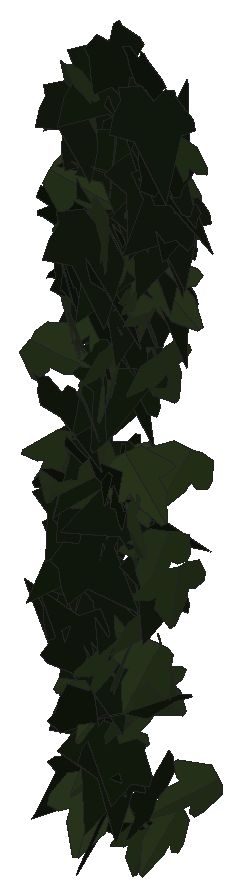
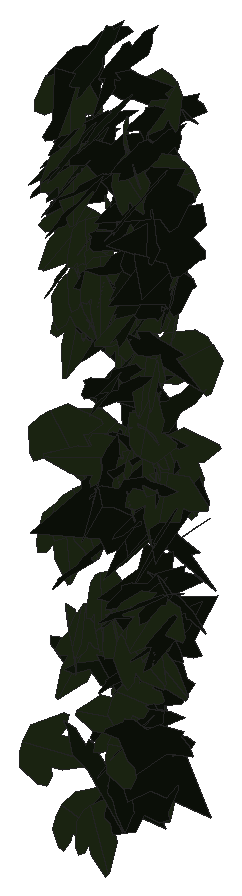
# SketchUp Ruby script. Lengths in inches.
U = 1.inch
M = Sketchup.active_model
def pt(a) = Geom::Point3d.new(a.map { |v| v * U })
def face(e, loops, mat)
  f = e.add_face(loops[0].map { |a| pt(a) })
  loops[1..].each { |l| e.add_face(l.map { |a| pt(a) }).erase! }
  f.material = f.back_material = mat if mat
  f
end
# faces: each face lists its corners as indices into pts; further lists are holes
def faces(e, pts, list, mat = nil) = list.each { |f| face(e, (f[0].is_a?(Array) ? f : [f]).map { |l| l.map { |i| pts[i] } }, mat) }
# xy, xz, yz: faces in a plane at the given z, y or x. An outline is a flat list of corners, or four numbers for a rectangle; further outlines are holes
def ring(l) = l.size == 4 ? [[l[0], l[1]], [l[2], l[1]], [l[2], l[3]], [l[0], l[3]]] : l.each_slice(2).to_a
def flat(e, list, mat, &to3) = list.each { |f| face(e, (f[0].is_a?(Array) ? f : [f]).map { |l| ring(l).map { |u, v| to3.(u, v) } }, mat) }
def xy(e, z, list, mat = nil) = flat(e, list, mat) { |x, y| [x, y, z] }
def xz(e, y, list, mat = nil) = flat(e, list, mat) { |x, z| [x, y, z] }
def yz(e, x, list, mat = nil) = flat(e, list, mat) { |y, z| [x, y, z] }
def lines(e, pts, list) = list.each { |a, b| e.add_line(pt(pts[a]), pt(pts[b])) }
# prism: a flat outline (further loops are holes) pulled along v
def prism(e, loops, v, mat = nil)
  f = face(e, loops, mat); d = Geom::Vector3d.new(v.map { |x| x * U })
  f.pushpull(f.normal.samedirection?(d) ? d.length : -d.length)
end
def box(e, o, s, mat = nil) = prism(e, [[o, [o[0] + s[0], o[1], o[2]], [o[0] + s[0], o[1] + s[1], o[2]], [o[0], o[1] + s[1], o[2]]]], [0, 0, s[2]], mat)
def at(x, y, z, deg = 0) = Geom::Transformation.translation(pt([x, y, z])) * Geom::Transformation.rotation(ORIGIN, Z_AXIS, deg.degrees)
def axes(o, x, y, z) = Geom::Transformation.new([*x, 0, *y, 0, *z, 0, *pt(o).to_a, 1])
def part(name) = M.definitions.add(name)
# library, detail: a bought-in or finely detailed component or shape, given as its bounding box
def library(name, o, s) = part(name).tap { |d| box(d.entities, o, s) }
def detail(e, o, s) = box(e.add_group.entities, o, s)
def put(e, d, t, mat = nil) = e.add_instance(d, t).tap { |i| i.material = mat if mat }
def group(e, t, mat = nil) = e.add_group.tap { |g| g.transformation = t; g.material = mat if mat }.entities
root = M.entities
M.materials.add("efeu1").color = [18, 25, 13]
M.materials.add("efeu2").color = [43, 57, 29]
c1 = part("ivyleaf_9")
p = [[1.54,2.16,1.25],[1.36,2.04,1.19],[-0.21,0.99,0.68],[-0.71,1.11,0.82],[-0.85,0.86,0.67],[-0.8,0.17,0.21],
  [-0.9,-0.01,0.1],[-0.67,-0.16,-0.02],[-0.08,-0.08,-0.05],[-0.03,-0.6,-0.4],[0.65,-0.88,-0.66],[0.83,-0.6,-0.49],
  [1.29,-0.42,-0.43],[1.8125,-0.07,-0.26],[1.21,0.44,0.15]]
faces(c1.entities,p,[[0,1,2,3,4,5,6,7,8,9,10,11,12,13,14]],"efeu1")
c2 = part("ivyleaf_10")
p = [[0,0.5,-0.03],[-0.0625,2.02,-0.43],[-0.19,2.01,-0.46],[-0.54,1.05,-0.29],[-0.52,0.625,-0.18],[-0.83,0.76,-0.28],
  [-1.16,0.64,-0.33],[-1.15,0.33,-0.24],[-0.77,-0.39,0.02],[-0.3,-0.51,0.16],[0.04,-0.48,0.23],[-0.02,2.01,-0.4375],
  [-0.06,2.01,-0.43],[0.04,-0.49,0.23],[0.67,-0.49,0.14],[1.38,0.36,-0.2],[1.375,0.51,-0.24],[0.81,0.65,-0.19],
  [0.62,0.59,-0.15],[0.6,1.09,-0.28],[0.5,1.23,-0.31]]
faces(c2.entities,p,[[0,1,2,3,4,5,6,7,8,9,10],[11,12,0,13,14,15,16,17,18,19,20]],"efeu2")
put(root,c1,axes([508.76,135.08,192.53],[-0.25978,-0.52817,0.37519],[0.04572,-0.39773,-0.57623],[0.68928,-0.17268,0.17963]))
put(root,c2,axes([509.12,134.49,194.79],[-0.36306,-0.7546,0.27247],[-0.10705,-0.25084,-0.83732],[0.79512,-0.37833,0.01169]))
put(root,c1,axes([509.24,135.42,198.38],[-0.72298,-0.08479,0.02489],[-0.02561,-0.00326,-0.70177],[0.09164,-0.66985,0.00027]))
put(root,c1,axes([508.4,134.64,201.28],[0.53749,0.06643,0.48148],[0.4958,0.05989,-0.52217],[-0.0966,0.67707,-0.00105]))
put(root,c2,axes([508.88,134.33,200.51],[-0.39697,0.64267,-0.05965],[0.0296,-0.0504,-0.76997],[-0.69621,-0.36859,0.00128]))
put(root,c1,axes([508.75,134.9,191.14],[-0.43366,-0.23224,-0.51261],[0.56748,-0.00304,-0.44369],[0.1557,-0.63574,0.18938]))
put(root,c1,axes([508.75,134.6875,190.26],[0.26594,-0.53794,-0.4122],[-0.15924,0.36824,-0.61506],[0.70385,0.28656,0.01659]))
put(root,c2,axes([508.62,134.04,197.67],[-0.37391,-0.21486,-0.64918],[0.609,0.27025,-0.42201],[0.37072,-0.66066,0.0385]))
put(root,c2,axes([509,134.86,194.03],[-0.62407,-0.48765,-0.09681],[0.19843,-0.07737,-0.76469],[0.4981,-0.58016,0.18335]))
put(root,c1,axes([508.88,134.89,199.27],[-0.02844,-0.15868,0.69998],[0.01988,-0.67347,-0.16438],[0.74657,0.01189,0.03104]))
put(root,c2,axes([509.25,134.22,198.74],[-0.59222,0.52666,0.21051],[-0.16923,0.129,-0.79057],[-0.58539,-0.57011,0.01558]))
put(root,c1,axes([509.17,134.29,194.01],[0.50767,0.49647,-0.21387],[-0.16249,-0.1407,-0.71094],[-0.55715,0.49341,0.01246]))
put(root,c1,axes([509.04,134.47,193.01],[0.40384,-0.34592,-0.49408],[-0.32095,0.37449,-0.52685],[0.54756,0.47463,0.05559]))
put(root,c2,axes([509.06,134.66,205.19],[-0.6331,0.3228,-0.21932],[0.20539,-0.09177,-0.69588],[-0.36225,-0.61618,-0.01125]))
put(root,c1,axes([509.14,134.65,199.38],[-0.13643,-0.25315,0.68709],[0.45043,0.51547,0.28835],[-0.61723,0.43213,0.05855]))
put(root,c2,axes([509.32,135.25,195.38],[-0.71365,0.12709,0.00293],[-0.00212,-0.02513,0.69933],[0.13728,0.66032,0.02606]))
put(root,c1,axes([509.03,134.41,200.02],[0.36968,0.37909,0.51686],[0.32165,0.39925,-0.53006],[-0.59351,0.4525,0.03467]))
put(root,c2,axes([509.14,135.05,190.63],[-0.59696,-0.24662,-0.30901],[0.3235,0.05357,-0.62576],[0.26318,-0.62525,0.06827]))
put(root,c1,axes([509.15,134.65,204.65],[-0.09175,-0.64913,-0.27211],[0.03492,0.25964,-0.68085],[0.75506,-0.09088,-0.00157]))
put(root,c1,axes([509.6875,134.27,192.35],[-0.79897,-0.00577,-0.06118],[0.06349,0.00497,-0.76939],[0.00664,-0.7421,-0.00467]))
put(root,c1,axes([508.85,134.5,196.1],[0.30426,-0.69778,0.23243],[0.26343,-0.13646,-0.76289],[0.74617,0.3327,0.17456]))
put(root,c1,axes([509.92,133.96,189.3],[0.14976,-0.00582,0.79224],[-0.72515,0.36482,0.13001],[-0.38864,-0.68295,0.0627]))
put(root,c2,axes([509.58,135,197.73],[-0.75329,0.2302,0.10623],[-0.12016,-0.03091,-0.78507],[-0.22325,-0.76012,0.0641]))
put(root,c1,axes([509.28,135.23,187.1875],[-0.3579,-0.4893,-0.43686],[0.3313,0.29581,-0.61004],[0.61262,-0.44582,0.07469]))
put(root,c1,axes([509.24,135.09,203.79],[0.23284,-0.66748,-0.43378],[-0.08207,0.42941,-0.70482],[0.79181,0.24079,0.0545]))
put(root,c2,axes([509.3,135.12,197.57],[-0.52207,0.38002,-0.45111],[0.29694,-0.3512,-0.6395],[-0.50965,-0.5939,0.08951]))
put(root,c1,axes([509.07,134.45,202.45],[0.70837,0.13278,0.28072],[0.28488,0.05738,-0.69596],[-0.15617,0.70694,0.00377]))
put(root,c1,axes([509.37,135.06,191.24],[-0.23069,-0.7832,-0.18856],[0.06214,0.17825,-0.81642],[0.80318,-0.23874,0.00901]))
put(root,c1,axes([509.35,135.33,192.45],[-0.15203,-0.63684,0.42663],[0.08409,-0.44617,-0.63605],[0.76191,-0.07783,0.15533]))
put(root,c2,axes([509.66,135.36,189.53],[0.00368,-0.66469,0.4371],[-0.02088,-0.43704,-0.66441],[0.79525,-0.0084,-0.01947]))
put(root,c2,axes([509.54,134.99,195.38],[0.70662,-0.37916,0.00544],[0.01402,0.01197,-0.78625],[0.40929,0.65419,0.01754]))
put(root,c2,axes([509.12,134.22,202.58],[-0.29437,-0.13343,-0.67628],[0.71205,0.02734,-0.29324],[0.08338,-0.70455,0.11669]))
put(root,c2,axes([510.18,134.26,188.82],[-0.48079,0.0072,0.64241],[-0.6439,-0.20429,-0.4444],[0.17462,-0.73348,0.13008]))
put(root,c1,axes([510.03,134.29,185.92],[0.0031,0.30802,-0.70925],[-0.23835,-0.65129,-0.3069],[-0.77222,0.20226,0.09187]))
put(root,c1,axes([510.05,135.15,205.34],[-0.77499,-0.18849,0.152],[-0.13731,-0.08975,-0.7696],[0.21794,-0.7268,0.05561]))
put(root,c2,axes([509.6875,134.39,196.18],[-0.5056,0.59976,0.04645],[-0.01629,0.04487,-0.79111],[-0.64933,-0.46813,-0.01632]))
put(root,c1,axes([509.53,135.47,190.71],[-0.26892,-0.68321,0.07895],[0.15285,-0.12997,-0.73363],[0.7265,-0.22555,0.18357]))
put(root,c1,axes([509.2,134.875,191.22],[0.60255,-0.30142,0.25891],[0.2394,-0.11343,-0.65948],[0.34777,0.60032,0.00539]))
put(root,c1,axes([509.45,135.36,189.04],[0.09907,-0.61465,0.23785],[0.05197,-0.224,-0.64616],[0.70638,0.10269,0.01418]))
put(root,c2,axes([509.8,135.4,202.9],[0.05303,-0.624,0.34407],[0.02217,-0.33023,-0.65095],[0.76246,0.053,-0.005]))
put(root,c1,axes([509.84,135.51,193.98],[-0.56027,-0.49969,-0.02015],[0.01249,0.01592,-0.74909],[0.53992,-0.51889,-0.00358]))
put(root,c1,axes([509.43,135.375,202.24],[0.28786,-0.76354,-0.00955],[0.00816,0.01328,-0.81591],[0.76356,0.28772,0.01232]))
put(root,c1,axes([509.87,135.52,196.8125],[-0.47167,-0.59525,0.19565],[-0.02059,-0.23003,-0.74949],[0.62625,-0.45589,0.12272]))
put(root,c2,axes([509.74,135.05,198.54],[0.39397,0.68512,-0.08166],[-0.03833,-0.07215,-0.79031],[-0.6889,0.39582,-0.00272]))
put(root,c1,axes([509.4,135.28,200.64],[0.05519,-0.13298,0.69325],[0.36607,-0.57444,-0.1462],[0.63631,0.34201,0.02398]))
put(root,c1,axes([509.61,134.63,193.12],[0.12573,-0.73854,-0.2323],[-0.00805,0.23409,-0.74857],[0.77417,0.12237,0.02994]))
put(root,c1,axes([510.1,134.75,195.03],[-0.69653,-0.35985,0.00332],[-0.00257,-0.00225,-0.78399],[0.35986,-0.69654,0.00082]))
put(root,c2,axes([510.03,135.04,187.79],[-0.29964,-0.35618,0.60833],[0.0521,-0.67039,-0.36685],[0.703,-0.10214,0.28647]))
put(root,c1,axes([509.85,135.3125,188.84],[-0.11584,-0.68495,0.21264],[0.0046,-0.20736,-0.72012],[0.77199,-0.10154,0.0362]))
put(root,c1,axes([509.65,134.6875,193.53],[-0.03226,0.11536,0.80072],[0.2664,-0.75515,0.11953],[0.76387,0.26823,-0.00787]))
put(root,c2,axes([510.05,134.38,193.68],[-0.64754,-0.60385,0.04266],[0.04023,0.01941,0.8853],[-0.60401,0.64865,0.01323]))
put(root,c2,axes([509.87,135.22,203.52],[0.44903,-0.39521,0.44386],[0.35811,-0.26998,-0.59596],[0.51614,0.53116,0.02734]))
put(root,c1,axes([509.8125,134,187.27],[-0.04821,-0.15599,0.76524],[0.71708,0.33816,0.11645],[-0.38168,0.65502,0.12213]))
put(root,c2,axes([510.21,135.02,186.29],[-0.0656,-0.34481,0.77559],[0.03401,-0.77835,-0.34315],[0.8481,0.00455,0.07375]))
put(root,c2,axes([510.09,134.09,185.41],[0.81443,0.29656,-0.10394],[-0.10024,-0.02849,-0.86671],[-0.29783,0.82054,0.00747]))
put(root,c2,axes([509.64,134.89,189.44],[0.23802,-0.3089,-0.7533],[0.57305,-0.49396,0.38362],[-0.57837,-0.61654,0.07008]))
put(root,c1,axes([509.96,135.02,206.26],[0.29331,-0.5605,-0.45763],[-0.2259,0.38746,-0.64754],[0.7357,0.34243,-0.01638]))
put(root,c1,axes([509.95,135.33,190.42],[-0.15664,-0.63717,0.38782],[0.11286,-0.41196,-0.63125],[0.73733,-0.07231,0.17901]))
put(root,c1,axes([509.81,134.52,198.99],[0.62133,-0.48941,-0.09932],[-0.07474,0.06604,-0.7855],[0.53332,0.57943,0.00564]))
put(root,c1,axes([510.04,134.35,201.34],[-0.29866,-0.70015,-0.37676],[0.12941,0.35429,-0.76097],[0.78448,-0.325,-0.01791]))
put(root,c1,axes([509.92,134.97,199.02],[0.67956,-0.38537,-0.15543],[-0.12265,0.09865,-0.78083],[0.39702,0.69009,0.02482]))
put(root,c1,axes([509.96,134.5625,184.4],[0.77428,0.13518,0.11322],[-0.12971,0.05233,0.75495],[0.13533,-0.72326,0.07579]))
put(root,c1,axes([509.8125,134.42,194.06],[-0.12829,-0.21871,0.75254],[0.54894,-0.56529,-0.09092],[0.6043,0.46707,0.24235]))
put(root,c1,axes([510.35,135.29,196.85],[-0.51768,-0.56878,0.02635],[-0.00704,-0.02764,-0.77346],[0.61485,-0.47921,0.01333]))
put(root,c2,axes([510.02,135.02,193.96],[0.30474,-0.43808,0.55132],[0.41807,-0.37243,-0.53437],[0.61388,0.4711,0.09024]))
put(root,c1,axes([510.11,133.68,192.57],[0.24357,-0.42772,-0.64861],[-0.18136,0.60624,-0.49556],[0.79635,0.26889,0.08553]))
put(root,c1,axes([510.45,134.92,200.82],[-0.57201,-0.5601,0.03966],[-0.00729,-0.0492,-0.8],[0.56146,-0.57127,0.03002]))
put(root,c2,axes([510.49,133.98,201.76],[0.56592,-0.46479,-0.38444],[-0.1681,0.38474,-0.7126],[0.57928,0.56571,0.16879]))
put(root,c2,axes([510.46,134.53,197.94],[-0.09696,-0.73812,-0.26175],[0.02212,0.25102,-0.77324],[0.84194,-0.0916,-0.00983]))
put(root,c1,axes([509.95,134.73,200.14],[0.44192,-0.64323,0.12152],[0.07484,-0.09439,-0.79281],[0.70208,0.41494,0.00803]))
put(root,c1,axes([510.15,134.41,189.49],[-0.37215,-0.40629,-0.56005],[0.45484,0.34281,-0.54925],[0.56913,-0.53964,0.07275]))
put(root,c1,axes([510.52,134.64,185.28],[-0.41059,0.29546,-0.63179],[0.44441,-0.45155,-0.49621],[-0.5786,-0.55649,0.0672]))
put(root,c1,axes([510.07,135.39,197.12],[0.39461,-0.68548,0.1194],[0.04902,-0.10953,-0.79086],[0.69408,0.39746,-0.01202]))
put(root,c1,axes([510.64,134.66,194.41],[0.21386,-0.05524,-0.82809],[-0.63582,0.53871,-0.20014],[0.53341,0.66428,0.09344]))
put(root,c2,axes([510.66,134.31,189.39],[-0.21816,-0.76009,0.09122],[-0.02477,-0.08466,-0.81793],[0.82597,-0.2033,-0.00043]))
put(root,c1,axes([510.59,134.45,186.69],[-0.48255,-0.63562,-0.03897],[0.02289,0.03091,-0.80802],[0.68728,-0.4473,-0.00045]))
put(root,c2,axes([510.52,134.7,186.84],[0.08193,-0.39193,0.68977],[-0.03294,0.6644,0.41194],[-0.83136,-0.06495,0.05166]))
put(root,c1,axes([510.46,135.14,203.38],[-0.33078,-0.6871,-0.27987],[0.12261,0.25158,-0.76258],[0.73171,-0.35277,0.00127]))
put(root,c1,axes([510.32,134.69,186.23],[0.08926,-0.75289,0.16921],[0.00504,-0.16315,-0.7876],[0.83188,0.08177,-0.01338]))
put(root,c1,axes([510.82,134.84,193.52],[-0.41237,-0.31937,0.57581],[-0.30118,-0.51268,-0.50005],[0.58553,-0.48863,0.14831]))
put(root,c1,axes([510.28,135.64,204.27],[0.07456,-0.65739,0.31488],[0.10468,-0.29301,-0.68462],[0.77462,0.10287,0.06221]))
put(root,c1,axes([511.29,134.63,198.38],[-0.18137,0.12053,0.79075],[-0.67534,0.41142,-0.21761],[-0.42863,-0.69922,0.00827]))
put(root,c2,axes([510.625,134.7,201.08],[0.7131,-0.37726,-0.01934],[-0.01708,0.00907,-0.80675],[0.37737,0.71331,0.00003]))
put(root,c2,axes([510.65,134.23,197.72],[0.55961,-0.55453,0.06624],[0.04571,-0.04762,-0.7893],[0.60109,0.51988,-0.00164]))
put(root,c2,axes([510.83,135.09,199.59],[-0.0617,-0.78049,-0.21693],[0.00006,0.21756,-0.78275],[0.81008,-0.05946,-0.01647]))
put(root,c2,axes([510.86,135.3125,184.13],[-0.11285,-0.71523,0.10454],[-0.00168,-0.10555,-0.72393],[0.72283,-0.11191,0.01464]))
put(root,c1,axes([510.67,135.12,199.87],[-0.23942,-0.77666,0.02771],[-0.00569,-0.02724,-0.81272],[0.77713,-0.23947,0.00258]))
put(root,c2,axes([510.91,134.43,189.54],[0.38124,-0.69875,-0.11774],[-0.06899,0.09455,-0.81403],[0.76137,0.35845,-0.01481]))
put(root,c1,axes([510.86,134.89,197.87],[-0.63445,-0.40163,-0.27007],[0.26293,0.08782,-0.74828],[0.40634,-0.68392,0.06251]))
put(root,c1,axes([510.4375,134.84,193.09],[0.71526,0.08674,0.40551],[0.40323,0.04329,-0.72049],[-0.09682,0.82108,-0.00486]))
put(root,c2,axes([511.13,134.68,190.34],[0.03198,-0.74517,-0.15737],[0.03451,0.15876,-0.74476],[0.76082,0.02412,0.0404]))
put(root,c1,axes([510.6875,135.32,205.85],[0.48165,-0.56595,0.08029],[0.03824,-0.07036,-0.74919],[0.6157,0.4471,-0.01628]))
put(root,c2,axes([511.13,134.875,199.08],[-0.55066,0.57233,-0.01593],[0.01171,-0.01085,-0.79422],[-0.57244,-0.55078,-0.00091]))
put(root,c1,axes([511.71,134.55,185.55],[-0.43157,0.66601,0.29854],[-0.16053,0.25171,-0.79361],[-0.71199,-0.46045,-0.00203]))
put(root,c2,axes([510.75,134.68,194.17],[0.15197,-0.12017,-0.83466],[0.74603,0.41455,0.07615],[0.39313,-0.74021,0.17815]))
put(root,c2,axes([511.4,135.49,199.15],[-0.18314,-0.71078,0.31527],[0.01884,-0.32786,-0.72822],[0.77734,-0.15952,0.09193]))
put(root,c2,axes([510.82,134.6,193.2],[-0.03862,0.06399,-0.86395],[0.56323,-0.65523,-0.07371],[-0.65823,-0.56442,-0.01238]))
put(root,c2,axes([511.4,135.07,199.43],[0.02533,-0.8054,0.11298],[0.00588,-0.11285,-0.80579],[0.81326,0.0259,0.00231]))
put(root,c2,axes([511.34,135.65,184.32],[-0.199,-0.48349,0.53658],[0.12004,-0.57097,-0.46996],[0.71223,-0.03885,0.22913]))
put(root,c1,axes([511.2,135.52,191.41],[-0.10856,-0.6919,0.29457],[0.03067,-0.30145,-0.69676],[0.75137,-0.08767,0.071]))
put(root,c2,axes([511.48,134.74,189.41],[-0.23517,-0.55927,0.45625],[0.04954,-0.49123,-0.57662],[0.72007,-0.14886,0.18868]))
put(root,c2,axes([511.06,134.47,194.8],[0.58902,0.26443,0.45486],[0.40176,0.23321,-0.62908],[-0.3785,0.65905,0.0401]))
put(root,c2,axes([511.58,134.72,200.23],[-0.0388,-0.78761,-0.13662],[0.03558,0.13494,-0.78805],[0.79857,-0.04428,0.02848]))
put(root,c2,axes([511.6875,134.96,192.67],[-0.36406,-0.64306,0.23922],[-0.05771,-0.24115,-0.73608],[0.68368,-0.36278,0.06525]))
put(root,c2,axes([511.68,135.15,202.49],[-0.40457,-0.7041,-0.01924],[0.06822,-0.01708,-0.80924],[0.70106,-0.40467,0.06764]))
put(root,c1,axes([511.5,135.24,201.75],[-0.27613,-0.73945,0.17309],[0.04301,-0.19911,-0.78199],[0.75822,-0.258,0.1074]))
put(root,c2,axes([511.6,134.65,188.63],[-0.29292,-0.52283,-0.46955],[0.2033,0.42391,-0.59883],[0.67268,-0.35578,-0.02349]))
put(root,c1,axes([511.375,135.34,201.53],[0.12907,-0.7895,0.08995],[0.01156,-0.08925,-0.79998],[0.79452,0.12955,-0.00298]))
put(root,c1,axes([511.67,134.85,203.24],[-0.30693,-0.75596,0.13747],[-0.00928,-0.14438,-0.81464],[0.7683,-0.30374,0.04508]))
put(root,c1,axes([511.36,135.4375,200.07],[0.31692,-0.79261,0.11744],[0.0234,-0.11709,-0.85335],[0.80092,0.31706,-0.02154]))
put(root,c2,axes([511.79,134.71,197.99],[-0.22534,-0.71646,-0.31183],[0.10747,0.29304,-0.75094],[0.77395,-0.24929,0.01348]))
put(root,c2,axes([512.04,135.37,194.97],[-0.54761,-0.42487,0.36354],[-0.20449,-0.32143,-0.68368],[0.52044,-0.57335,0.11389]))
put(root,c1,axes([511.41,134.8,188.1],[-0.33705,-0.70874,0.01266],[0.7561,-0.31027,-0.12064],[0.11991,-0.03574,0.7963]))
put(root,c2,axes([512.1,134.85,204.26],[-0.80672,-0.03071,0.18719],[-0.18703,-0.00769,-0.80731],[0.03165,-0.82812,0.00056]))
put(root,c1,axes([511.48,135.2,203.15],[0.5169,-0.63502,-0.09522],[0.00904,0.12942,-0.81405],[0.64206,0.50942,0.08812]))
put(root,c1,axes([511.58,135.33,202.22],[-0.00253,-0.63401,0.51191],[0.15875,-0.50249,-0.62156],[0.79926,0.09779,0.12507]))
put(root,c2,axes([511.49,135.29,188.8],[-0.20185,0.06171,0.76413],[0.66326,-0.38217,0.20607],[0.38442,0.69179,0.04568]))
put(root,c1,axes([511.59,135.25,202.1],[0.21888,-0.77694,0.1094],[0.02534,-0.10651,-0.80717],[0.78419,0.2203,-0.00445]))
put(root,c1,axes([511.74,135.25,202.43],[0.05763,-0.81127,-0.0914],[0.01434,0.09262,-0.81305],[0.81628,0.05565,0.02073]))
put(root,c1,axes([512.11,134.53,203.45],[-0.21695,-0.36537,0.7381],[0.38244,0.6313,0.42491],[-0.7294,0.43968,0.00326]))
put(root,c1,axes([511.8,134.4,205.44],[0.02238,-0.83273,-0.14823],[0.01877,0.14874,-0.83273],[0.84561,0.01874,0.02241]))
put(root,c2,axes([512.24,134.77,191.99],[-0.28838,-0.76413,-0.00461],[0.00051,0.00474,-0.81674],[0.76414,-0.28838,-0.0012]))
put(root,c1,axes([512.15,134.92,202.62],[-0.30386,-0.56755,0.50605],[-0.16,-0.48503,-0.64006],[0.74337,-0.33639,0.06909]))
put(root,c2,axes([511.91,134.5,200.4],[-0.48255,-0.46285,-0.4604],[0.47498,0.14385,-0.64246],[0.44787,-0.65125,0.1853]))
put(root,c2,axes([512.47,135.57,185.76],[-0.09897,-0.2883,0.69705],[-0.25509,-0.64882,-0.30457],[0.70988,-0.27334,-0.01226]))
